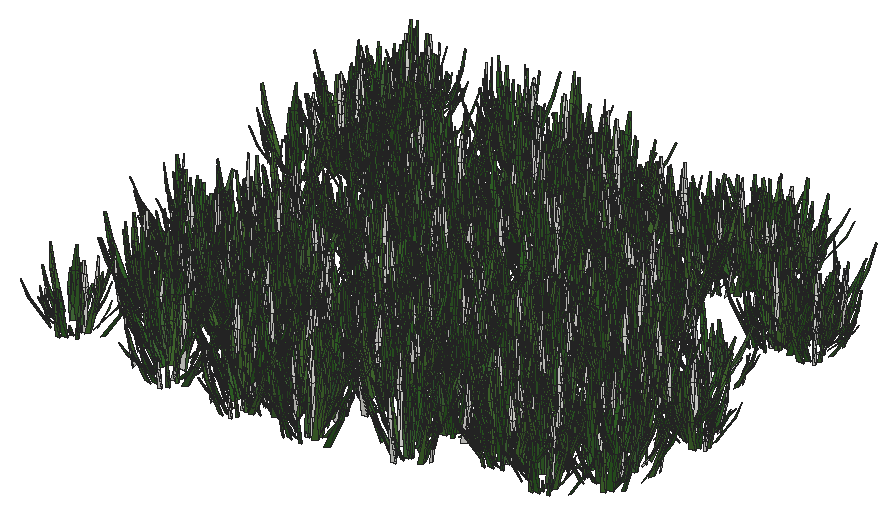
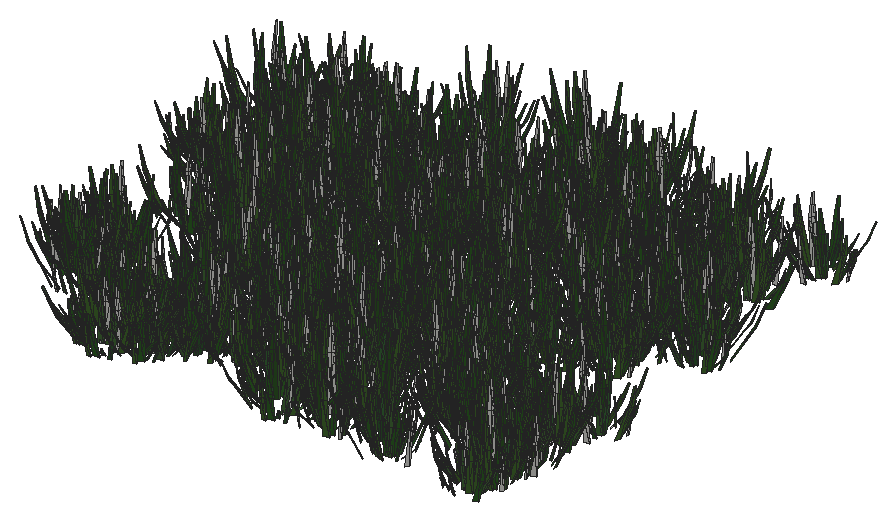
# SketchUp Ruby script. Lengths in inches.
U = 1.inch
M = Sketchup.active_model
def pt(a) = Geom::Point3d.new(a.map { |v| v * U })
def face(e, loops, mat)
  f = e.add_face(loops[0].map { |a| pt(a) })
  loops[1..].each { |l| e.add_face(l.map { |a| pt(a) }).erase! }
  f.material = f.back_material = mat if mat
  f
end
# faces: each face lists its corners as indices into pts; further lists are holes
def faces(e, pts, list, mat = nil) = list.each { |f| face(e, (f[0].is_a?(Array) ? f : [f]).map { |l| l.map { |i| pts[i] } }, mat) }
# xy, xz, yz: faces in a plane at the given z, y or x. An outline is a flat list of corners, or four numbers for a rectangle; further outlines are holes
def ring(l) = l.size == 4 ? [[l[0], l[1]], [l[2], l[1]], [l[2], l[3]], [l[0], l[3]]] : l.each_slice(2).to_a
def flat(e, list, mat, &to3) = list.each { |f| face(e, (f[0].is_a?(Array) ? f : [f]).map { |l| ring(l).map { |u, v| to3.(u, v) } }, mat) }
def xy(e, z, list, mat = nil) = flat(e, list, mat) { |x, y| [x, y, z] }
def xz(e, y, list, mat = nil) = flat(e, list, mat) { |x, z| [x, y, z] }
def yz(e, x, list, mat = nil) = flat(e, list, mat) { |y, z| [x, y, z] }
def lines(e, pts, list) = list.each { |a, b| e.add_line(pt(pts[a]), pt(pts[b])) }
# prism: a flat outline (further loops are holes) pulled along v
def prism(e, loops, v, mat = nil)
  f = face(e, loops, mat); d = Geom::Vector3d.new(v.map { |x| x * U })
  f.pushpull(f.normal.samedirection?(d) ? d.length : -d.length)
end
def box(e, o, s, mat = nil) = prism(e, [[o, [o[0] + s[0], o[1], o[2]], [o[0] + s[0], o[1] + s[1], o[2]], [o[0], o[1] + s[1], o[2]]]], [0, 0, s[2]], mat)
def at(x, y, z, deg = 0) = Geom::Transformation.translation(pt([x, y, z])) * Geom::Transformation.rotation(ORIGIN, Z_AXIS, deg.degrees)
def axes(o, x, y, z) = Geom::Transformation.new([*x, 0, *y, 0, *z, 0, *pt(o).to_a, 1])
def part(name) = M.definitions.add(name)
# library, detail: a bought-in or finely detailed component or shape, given as its bounding box
def library(name, o, s) = part(name).tap { |d| box(d.entities, o, s) }
def detail(e, o, s) = box(e.add_group.entities, o, s)
def put(e, d, t, mat = nil) = e.add_instance(d, t).tap { |i| i.material = mat if mat }
def group(e, t, mat = nil) = e.add_group.tap { |g| g.transformation = t; g.material = mat if mat }.entities
root = M.entities
M.materials.add("Material1").color = [58, 110, 58]
M.materials.add("Material10").color = [48, 100, 38]
M.materials.add("Material3").color = [68, 110, 58]
M.materials.add("Material4").color = [48, 90, 38]
M.materials.add("Material5").color = [68, 110, 48]
M.materials.add("Material6").color = [48, 90, 48]
M.materials.add("Material8").color = [58, 90, 38]
M.materials.add("Material9").color = [68, 100, 58]
c1 = part("grass00")
p = [[-0.6875,0.15,0],[-0.56,0.08,5.52],[-0.04,0.03,2.76],[0.48,-0.02,0],[0.35,-0.02,5.52],[-0.1,-0.14,5.52],
  [-0.12,0.65,8.37],[-0.42,0.65,8.37]]
faces(c1.entities,p,[[0,1,2,3],[3,2,4],[1,5,2],[5,4,2],[1,6,5],[4,5,6],[7,6,1]])
c2 = part("Group16\#1")
put(c2.entities,c1,axes([1.44,-0.61,-0.01],[0.05352,0.12609,0],[-0.10704,0.04543,0.07239],[0.06664,-0.02828,0.11628]),"Material6")
put(c2.entities,c1,axes([0.76,-0.15,-0.01],[0.04676,0.24062,0],[-0.23162,0.04501,0.06642],[0.0652,-0.01267,0.23595]),"Material3")
put(c2.entities,c1,axes([0.79,0.01,-0.01],[-0.00606,0.34651,0],[-0.34381,-0.00602,0.0432],[0.04319,0.00076,0.34386]))
put(c2.entities,c1,axes([1,0.23,-0.01],[-0.07192,0.31144,0],[-0.28722,-0.06632,0.1236],[0.12043,0.02781,0.29478]),"Material5")
put(c2.entities,c1,axes([1.66,0.77,-0.01],[-0.13828,0.29651,0],[-0.21551,-0.1005,0.22471],[0.20365,0.09498,0.23779]),"Material10")
put(c2.entities,c1,axes([0.6875,0.52,-0.01],[-0.18126,0.24051,0],[-0.22746,-0.17142,0.09788],[0.07817,0.05891,0.28481]),"Material5")
put(c2.entities,c1,axes([0.68,0.78,-0.01],[-0.215,0.18688,0],[-0.12385,-0.14248,0.21334],[0.13995,0.16101,0.18878]),"Material3")
put(c2.entities,c1,axes([0.56,1,-0.01],[-0.13756,0.07624,0],[-0.06159,-0.11112,0.0927],[0.04494,0.08108,0.12705]),"Material5")
put(c2.entities,c1,axes([0.2,0.64,-0.01],[-0.23729,0.07254,0],[-0.05711,-0.18681,0.153],[0.04473,0.14632,0.19535]),"Material10")
put(c2.entities,c1,axes([0.0625,0.72,-0.01],[-0.28874,0.02525,0],[-0.02179,-0.24916,0.14647],[0.01276,0.14591,0.25012]),"Material3")
put(c2.entities,c1,axes([-0.08,0.62,-0.01],[-0.34089,-0.04187,0],[0.03255,-0.26504,0.216],[-0.02633,0.21439,0.26703]),"Material10")
put(c2.entities,c1,axes([-0.34,0.98,-0.01],[-0.14314,-0.0493,0],[0.04397,-0.12769,0.06843],[-0.02228,0.0647,0.13505]),"Material10")
put(c2.entities,c1,axes([-0.87,1.45,-0.01],[-0.23488,-0.14114,0],[0.13761,-0.22901,0.06087],[-0.03135,0.05217,0.26717]))
put(c2.entities,c1,axes([-0.72,0.77,-0.01],[-0.14208,-0.13251,0],[0.07209,-0.0773,0.16301],[-0.11118,0.11922,0.1057]),"Material10")
put(c2.entities,c1,axes([-0.62,0.43,-0.01],[-0.14845,-0.21203,0],[0.18654,-0.13061,0.12304],[-0.10079,0.07057,0.22772]),"Material3")
put(c2.entities,c1,axes([-0.68,0.29,-0.01],[-0.13639,-0.32136,0],[0.31723,-0.13464,0.05579],[-0.05136,0.0218,0.34462]),"Material4")
put(c2.entities,c1,axes([-0.64,0.125,-0.01],[-0.0458,-0.23569,0],[0.22124,-0.043,0.08276],[-0.08124,0.01579,0.22538]),"Material1")
put(c2.entities,c1,axes([-1.6,-0.03,-0.01],[0.00576,-0.32897,0],[0.27526,0.00482,0.18018],[-0.18015,-0.00315,0.2753]),"Material5")
put(c2.entities,c1,axes([-1.36,-0.31,-0.01],[0.05718,-0.24765,0],[0.18172,0.04196,0.17267],[-0.16825,-0.03885,0.1865]),"Material10")
put(c2.entities,c1,axes([-1.54,-0.72,-0.01],[0.06537,-0.14017,0],[0.13555,0.06321,0.03939],[-0.0357,-0.01665,0.14956]))
put(c2.entities,c1,axes([-1.19,-0.9,-0.01],[0.09597,-0.12735,0],[0.11214,0.08451,0.07557],[-0.06035,-0.04548,0.14042]),"Material9")
put(c2.entities,c1,axes([-0.47,-0.54,-0.01],[0.11588,-0.10072,0],[0.0618,0.0711,0.12124],[-0.07953,-0.0915,0.0942]))
put(c2.entities,c1,axes([-0.47,-0.84,-0.01],[0.11927,-0.0661,0],[0.06603,0.11913,0.00646],[-0.00313,-0.00565,0.13621]),"Material5")
put(c2.entities,c1,axes([-0.38,-1.24,-0.01],[0.28037,-0.08571,0],[0.0618,0.20215,0.20315],[-0.05939,-0.19428,0.21139]),"Material9")
put(c2.entities,c1,axes([-0.06,-0.66,-0.01],[0.22719,-0.01987,0],[0.01247,0.14255,0.17758],[-0.01547,-0.17691,0.1431]),"Material8")
put(c2.entities,c1,axes([0.11,-0.89,-0.01],[0.14882,0.01828,0],[-0.01058,0.08611,0.12229],[0.01491,-0.12138,0.08676]),"Material6")
put(c2.entities,c1,axes([0.25,-0.72,-0.01],[0.20481,0.07053,0],[-0.06206,0.18022,0.10291],[0.03351,-0.0973,0.1906]),"Material6")
put(c2.entities,c1,axes([0.85,-1.42,-0.01],[0.16481,0.09904,0],[-0.09472,0.15762,0.05616],[0.02893,-0.04814,0.18389]),"Material5")
put(c2.entities,c1,axes([1.01,-1.09,-0.01],[0.21858,0.20385,0],[-0.17495,0.1876,0.15339],[0.10462,-0.11218,0.25652]),"Material10")
put(c2.entities,c1,axes([1.01,-0.71,-0.01],[0.08733,0.12473,0],[-0.06445,0.04512,0.13037],[0.1068,-0.07477,0.07867]),"Material6")
c3 = part("Group15\#1")
put(c3.entities,c2,at(0,0,0))
c4 = part("3darcstudiotree_grass00\#1")
put(c4.entities,c3,at(0,0,0))
put(root,c4,axes([316.35,97.13,0.25],[0.80132,-0.79526,0],[0.85381,0.59267,-0.02296],[0.02904,0.02016,1.8355]))
put(root,c4,axes([311.95,97.03,0.25],[0.12403,0.97719,0],[-0.92314,0.08072,-0.01763],[-0.03038,0.00266,1.60818]))
put(root,c4,axes([306.93,97.28,0.25],[0.20724,0.95588,0],[-1.27061,0.18977,-0.03105],[-0.03558,0.00531,1.50318]))
put(root,c4,axes([299.84,98.125,0.25],[0.90774,-0.36682,0],[0.49789,0.84879,-0.02466],[0.01422,0.02424,1.49812]))
put(root,c4,axes([313.64,97.92,0.25],[0.71273,0.60572,0],[-0.70706,0.57314,-0.01838],[-0.02206,0.01788,1.65818]))
put(root,c4,axes([321.96,98.48,0.25],[-0.85719,0.37482,0],[-0.44623,-0.70302,-0.01732],[-0.0161,-0.02536,1.90951]))
put(root,c4,axes([305.42,99.13,0.25],[1.00849,0.25736,0],[-0.35211,0.95054,-0.02064],[-0.00744,0.02009,1.46981]))
put(root,c4,axes([310.03,99.36,0.25],[0.41909,-0.86527,0],[1.14973,0.38363,-0.01772],[0.02372,0.00791,1.7874]))
put(root,c4,axes([315.09,99.53,0.25],[-0.98897,0.46793,0],[-0.61487,-0.89525,-0.01918],[-0.01379,-0.02007,1.80194]))
put(root,c4,axes([329.375,100.51,0.25],[1.05308,-0.43732,0],[0.41642,0.6908,-0.01525],[0.01172,0.01944,1.59832]))
put(root,c4,axes([326.36,101.1875,0.25],[0.78883,-0.48342,0],[0.67697,0.76099,-0.02283],[0.01727,0.01941,1.4512]))
put(root,c4,axes([303.67,101.62,0.25],[1.18479,-0.24576,0],[0.30744,1.02105,-0.03338],[0.00879,0.02919,1.37691]))
put(root,c4,axes([321.91,101.61,0.25],[-1.05079,-0.61219,0],[0.56436,-0.66733,-0.02484],[0.02413,-0.02854,1.66133]))
put(root,c4,axes([308.4375,101.85,0.25],[1.16137,-0.01703,0],[0.0221,1.03814,-0.02875],[0.00063,0.02974,1.55972]))
put(root,c4,axes([303.02,101.74,0.25],[-0.72355,-0.65418,0],[0.95278,-0.72597,-0.02326],[0.02414,-0.01839,1.82249]))
put(root,c4,axes([313.32,101.96,0.25],[0.32014,-0.85505,0],[1.06307,0.2742,-0.02169],[0.02869,0.0074,1.54236]))
put(root,c4,axes([325.75,102.07,0.25],[1.03078,-0.2005,0],[0.29521,1.04552,-0.02268],[0.00619,0.02191,1.5468]))
put(root,c4,axes([317.88,101.84,0.25],[-0.934,0.44634,0],[-0.64253,-0.92624,-0.0199],[-0.01289,-0.01859,1.67187]))
put(root,c4,axes([311.94,102.48,0.25],[-0.6646,-0.67167,0],[0.74435,-0.50738,-0.021],[0.02364,-0.01611,1.40308]))
put(root,c4,axes([301.47,102.32,0.25],[-0.81371,0.66575,0],[-0.86342,-0.727,-0.01243],[-0.01253,-0.01055,1.76595]))
put(root,c4,axes([331.54,102.84,0.25],[1.28074,0.0617,0],[-0.0694,0.99245,-0.0212],[-0.00202,0.02883,1.96575]))
put(root,c4,axes([324.94,103.13,0.25],[0.07007,-0.79845,0],[0.91239,0.05516,-0.00937],[0.0198,0.0012,1.93766]))
put(root,c4,axes([319.48,103.07,0.25],[-0.36362,-0.73138,0],[1.12762,-0.38622,-0.01762],[0.01979,-0.00678,1.48208]))
put(root,c4,axes([327.05,102.92,0.25],[-0.4787,0.65235,0],[-0.88098,-0.44536,-0.03041],[-0.03325,-0.01681,1.3205]))
put(root,c4,axes([308.77,103.05,0.25],[-1.08604,-0.15157,0],[0.17672,-0.87228,-0.0114],[0.0035,-0.01728,1.97478]))
put(root,c4,axes([328.02,103.05,0.25],[-0.16041,0.91007,0],[-0.94249,-0.11444,-0.02144],[-0.04347,-0.00528,1.9513]))
put(root,c4,axes([304.47,103.25,0.25],[-0.94592,0.10903,0],[-0.1657,-0.99036,-0.02154],[-0.00353,-0.02108,1.4342]))
put(root,c4,axes([313.27,103.47,0.25],[-0.88718,-0.16403,0],[0.21188,-0.78948,-0.02543],[0.00915,-0.03409,1.61262]))
put(root,c4,axes([317.96,104.16,0.25],[0.65668,-0.79697,0],[0.79285,0.45005,-0.02882],[0.03521,0.01999,1.42183]))
put(root,c4,axes([322.01,104.29,0.25],[1.1345,0.2801,0],[-0.33208,0.9266,-0.03162],[-0.0104,0.02903,1.3441]))
put(root,c4,axes([302.77,104.28,0.25],[0.93252,0.18888,0],[-0.22324,0.75929,-0.01459],[-0.00645,0.02194,1.75568]))
put(root,c4,axes([315.06,104.44,0.25],[1.27135,0.10554,0],[-0.11776,0.97731,-0.02551],[-0.00318,0.02637,1.48132]))
put(root,c4,axes([305.96,104.14,0.25],[-0.95929,-0.15943,0],[0.24233,-1.00448,-0.02406],[0.00588,-0.02436,1.53532]))
put(root,c4,axes([304.3,104.21,0.25],[0.36677,0.87584,0],[-0.8672,0.25018,-0.01128],[-0.02111,0.00609,1.81963]))
put(root,c4,axes([316.33,104.4,0.25],[0.63898,0.91689,0],[-1.0111,0.48542,-0.02506],[-0.03395,0.0163,1.82822]))
put(root,c4,axes([308.27,104.79,0.25],[-0.23441,-0.84252,0],[0.89566,-0.17167,-0.0292],[0.04766,-0.00914,1.53984]))
put(root,c4,axes([331.91,104.58,0.25],[-1.08025,0.12081,0],[-0.14812,-0.9124,-0.01091],[-0.00245,-0.01509,1.8656]))
put(root,c4,axes([311.97,104.98,0.25],[-1.17861,0.11572,0],[-0.13809,-0.96888,-0.02284],[-0.00331,-0.0232,1.44864]))
put(root,c4,axes([309.13,105.45,0.25],[-0.68321,-0.72872,0],[0.78352,-0.50606,-0.01663],[0.02499,-0.01614,1.89037]))
put(root,c4,axes([328.33,105.7,0.25],[0.40907,-0.67881,0],[0.97262,0.40378,-0.01805],[0.02352,0.00976,1.58457]))
put(root,c4,axes([303.86,105.63,0.25],[0.86846,0.22562,0],[-0.28927,0.76707,-0.01935],[-0.01148,0.03043,1.92273]))
put(root,c4,axes([322.75,105.79,0.25],[0.97724,-0.26245,0],[0.36108,0.9262,-0.01717],[0.0067,0.0172,1.48777]))
put(root,c4,axes([319.73,105.9,0.25],[0.96998,-0.05804,0],[0.06668,0.76779,-0.00836],[0.00128,0.01473,1.97523]))
put(root,c4,axes([316.75,105.83,0.25],[0.12117,0.83819,0],[-0.93224,0.09284,-0.01784],[-0.034,0.00339,1.80168]))
put(root,c4,axes([309.8125,105.86,0.25],[0.04694,1.0652,0],[-1.26088,0.03828,-0.0182],[-0.02086,0.00063,1.44668]))
put(root,c4,axes([326.38,106.08,0.25],[-0.28901,0.78465,0],[-1.0714,-0.27186,-0.0271],[-0.04002,-0.01015,1.72974]))
put(root,c4,axes([305.92,106.65,0.25],[0.07107,0.86763,0],[-1.08123,0.06101,-0.02807],[-0.03406,0.00192,1.3177]))
put(root,c4,axes([325.18,106.91,0.25],[-1.06982,0.08364,0],[-0.10313,-0.90868,-0.0202],[-0.00337,-0.02969,1.95637]))
put(root,c4,axes([317.59,107.38,0.25],[0.86287,-0.53565,0],[0.7402,0.82143,-0.02614],[0.01879,0.02086,1.48366]))
put(root,c4,axes([300.78,107.27,0.25],[1.16448,0.38507,0],[-0.42835,0.89237,-0.01606],[-0.00795,0.01656,1.54782]))
put(root,c4,axes([330.03,107.22,0.25],[0.60099,0.7227,0],[-0.87959,0.5039,-0.02215],[-0.0291,0.01667,1.70619]))
put(root,c4,axes([318.74,107.37,0.25],[-0.84677,-0.53059,0],[0.70417,-0.77417,-0.01411],[0.01233,-0.01356,1.69584]))
put(root,c4,axes([308.43,107.44,0.25],[-0.07251,0.86254,0],[-1.06517,-0.06169,-0.02357],[-0.034,-0.00197,1.54387]))
put(root,c4,axes([299.66,107.88,0.25],[0.62341,-0.65045,0],[0.81136,0.53571,-0.01848],[0.02058,0.01359,1.47553]))
put(root,c4,axes([320.87,108.25,0.25],[0.32381,0.70798,0],[-1.1928,0.37583,-0.02635],[-0.03281,0.01034,1.69955]))
put(root,c4,axes([316.57,108.31,0.25],[0.65479,0.79637,0],[-0.75973,0.43034,-0.01403],[-0.02494,0.01413,1.97952]))
put(root,c4,axes([313.28,108.45,0.25],[-0.31977,-0.73816,0],[0.97929,-0.29225,-0.0171],[0.02773,-0.00828,1.79343]))
put(root,c4,axes([312.07,108.25,0.25],[0.23878,1.03245,0],[-1.19555,0.19048,-0.02457],[-0.03165,0.00504,1.59681]))
put(root,c4,axes([303.11,108.54,0.25],[-0.25504,0.90723,0],[-0.99851,-0.19338,-0.02125],[-0.02713,-0.00525,1.34411]))
put(root,c4,axes([305.28,108.6,0.25],[-0.52673,0.64023,0],[-0.75004,-0.4251,-0.01899],[-0.03039,-0.01722,1.75992]))
put(root,c4,axes([323.56,109.13,0.25],[1.0339,-0.45076,0],[0.45476,0.71859,-0.02304],[0.01955,0.0309,1.78453]))
put(root,c4,axes([321.25,109.39,0.25],[0.04633,-0.80855,0],[0.9767,0.03855,-0.0123],[0.02217,0.00088,1.7643]))
put(root,c4,axes([317.79,109.36,0.25],[-0.28741,-0.72638,0],[0.96366,-0.26268,-0.02104],[0.0287,-0.00782,1.45661]))
put(root,c4,axes([332.67,109.11,0.25],[-0.50829,0.70684,0],[-0.88646,-0.43915,-0.0186],[-0.02272,-0.01125,1.46845]))
put(root,c4,axes([299.2,109.625,0.25],[-1.10338,-0.30687,0],[0.31079,-0.76983,-0.02118],[0.01148,-0.02843,1.66873]))
put(root,c4,axes([331.375,109.95,0.25],[-0.28588,-0.97039,0],[1.21013,-0.2456,-0.03172],[0.03382,-0.00686,1.36741]))
put(root,c4,axes([327.19,109.6875,0.25],[-0.19365,0.85401,0],[-1.21133,-0.18922,-0.01956],[-0.02828,-0.00442,1.8138]))
put(root,c4,axes([311.23,109.73,0.25],[-0.46557,0.88149,0],[-0.85697,-0.31181,-0.01229],[-0.02382,-0.00867,1.9803]))
put(root,c4,axes([316.24,110.5,0.25],[1.27169,-0.1612,0],[0.14546,0.79054,-0.02943],[0.00699,0.03801,1.51666]))
put(root,c4,axes([326.95,110.93,0.25],[-0.95819,-0.35748,0],[0.36939,-0.68208,-0.02079],[0.01525,-0.02816,1.61237]))
put(root,c4,axes([305.45,110.91,0.25],[-1.11893,-0.19294,0],[0.25521,-1.01964,-0.02537],[0.00751,-0.03001,1.82613]))
put(root,c4,axes([328.55,111.28,0.25],[0.57634,-0.70266,0],[0.90577,0.51181,-0.01892],[0.02488,0.01406,1.74337]))
put(root,c4,axes([323.92,111.11,0.25],[0.80339,0.50827,0],[-0.58384,0.63574,-0.01463],[-0.01601,0.01743,1.73802]))
put(root,c4,axes([317.8,110.97,0.25],[-1.24958,0.10274,0],[-0.09107,-0.76308,-0.0174],[-0.0032,-0.02684,1.72585]))
put(root,c4,axes([302.15,111.21,0.25],[-0.54044,-0.83323,0],[0.96155,-0.42964,-0.02018],[0.03177,-0.01419,1.95264]))
put(root,c4,axes([320.93,111.87,0.25],[0.88102,0.19888,0],[-0.2921,0.89141,-0.02379],[-0.00841,0.02566,1.49895]))
put(root,c4,axes([311.74,111.98,0.25],[0.91654,0.42489,0],[-0.49728,0.73898,-0.02091],[-0.01555,0.02311,1.55496]))
put(root,c4,axes([303.62,111.8125,0.25],[-0.78623,0.83967,0],[-0.77178,-0.49784,-0.03149],[-0.03404,-0.02196,1.33797]))
put(root,c4,axes([321.875,112.1,0.25],[0.58794,0.7169,0],[-0.77809,0.43961,-0.02533],[-0.03533,0.01996,1.58831]))
put(root,c4,axes([324.26,112.26,0.25],[0.92637,0.60353,0],[-0.62404,0.65986,-0.02005],[-0.0228,0.02411,1.86077]))
put(root,c4,axes([326.75,112.17,0.25],[-0.61592,0.73394,0],[-0.79423,-0.45916,-0.01437],[-0.02338,-0.01352,1.91898]))
put(root,c4,axes([312.96,112.51,0.25],[-0.69305,-0.66666,0],[0.88309,-0.63244,-0.03179],[0.0275,-0.01969,1.33245]))
put(root,c4,axes([302.39,112.93,0.25],[0.8253,-0.5081,0],[0.63121,0.70631,-0.02804],[0.02455,0.02747,1.55696]))
put(root,c4,axes([321.98,113.01,0.25],[0.58294,0.61529,0],[-0.97292,0.635,-0.01217],[-0.01408,0.00919,1.82194]))
put(root,c4,axes([319.36,113.43,0.25],[1.20286,-0.08126,0],[0.0966,0.98504,-0.02372],[0.0024,0.02445,1.48337]))
put(root,c4,axes([307.25,113.15,0.25],[-0.95152,-0.19631,0],[0.29747,-0.99332,-0.01735],[0.00577,-0.01928,1.70162]))
put(root,c4,axes([317.95,113.44,0.25],[1.03718,0.55321,0],[-0.70077,0.90509,-0.03131],[-0.01945,0.02512,1.48921]))
put(root,c4,axes([314.17,113.61,0.25],[-0.70254,0.68427,0],[-0.92407,-0.65358,-0.01912],[-0.01621,-0.01147,1.35238]))
put(root,c4,axes([312.12,113.72,0.25],[-0.97108,0.42527,0],[-0.49629,-0.7807,-0.01893],[-0.01139,-0.01792,1.37131]))
put(root,c4,axes([315.07,114.3125,0.25],[-0.10669,0.80768,0],[-1.01448,-0.09232,-0.02456],[-0.04084,-0.00372,1.70727]))
put(root,c4,axes([305.27,114.47,0.25],[-1.01459,-0.57502,0],[0.51409,-0.62489,-0.01838],[0.02057,-0.025,1.80866]))
put(root,c4,axes([329.32,114.73,0.25],[-1.14951,0.07107,0],[-0.07117,-0.79306,-0.0204],[-0.00216,-0.02409,1.3669]))
put(root,c4,axes([309.68,114.86,0.25],[-1.00145,-0.49535,0],[0.54618,-0.7607,-0.01663],[0.01553,-0.02163,1.94585]))
put(root,c4,axes([320.8,114.99,0.25],[-0.59135,0.86757,0],[-0.96172,-0.45159,-0.02589],[-0.02858,-0.01342,1.40149]))
put(root,c4,axes([324.91,115.6,0.25],[-0.35506,-0.69296,0],[1.04061,-0.36732,-0.01791],[0.02769,-0.00977,1.89984]))
put(root,c4,axes([310.39,115.61,0.25],[-1.10357,-0.1539,0],[0.16872,-0.83348,-0.01654],[0.00511,-0.02523,1.89711]))
put(root,c4,axes([306.85,115.91,0.25],[0.53466,0.61624,0],[-0.7851,0.46925,-0.02117],[-0.0301,0.01799,1.69559]))
put(root,c4,axes([316.21,117.12,0.25],[1.01453,-0.24669,0],[0.31532,0.89333,-0.01036],[0.00503,0.01424,1.93559]))
put(root,c4,axes([308.36,116.89,0.25],[0.55253,0.95891,0],[-0.94558,0.37535,-0.02212],[-0.03718,0.01476,1.95299]))
put(root,c4,axes([312.83,117.13,0.25],[-0.83676,-0.36548,0],[0.46586,-0.73476,-0.01604],[0.0142,-0.0224,1.9024]))
put(root,c4,axes([322.05,117.04,0.25],[-0.41283,0.85285,0],[-1.03697,-0.3458,-0.02547],[-0.02931,-0.00978,1.38631]))
put(root,c4,axes([323.68,117.32,0.25],[-0.75666,-0.75068,0],[0.85742,-0.59539,-0.01878],[0.02166,-0.01504,1.68146]))
put(root,c4,axes([323.67,117.93,0.25],[-1.1416,0.45714,0],[-0.45611,-0.78467,-0.02532],[-0.01721,-0.02961,1.64221]))
put(root,c4,axes([311.72,118.4,0.25],[1.15172,0.48664,0],[-0.57188,0.9324,-0.01612],[-0.0094,0.01532,1.61949]))
put(root,c4,axes([298.58,118.59,0.25],[1.04476,-0.17024,0],[0.22274,0.94168,-0.02697],[0.00719,0.03039,1.59996]))
put(root,c4,axes([305.64,118.59,0.25],[1.14989,-0.07767,0],[0.09108,0.92892,-0.01977],[0.00228,0.02329,1.59866]))
put(root,c4,axes([315.29,118.28,0.25],[-1.09908,0.39917,0],[-0.45844,-0.86957,-0.02625],[-0.01345,-0.02552,1.46233]))
put(root,c4,axes([313.1,119.18,0.25],[0.11479,-0.84282,0],[1.27851,0.11996,-0.01256],[0.01851,0.00174,1.90836]))
put(root,c4,axes([329.55,119.66,0.25],[0.60422,-0.56041,0],[0.75524,0.56096,-0.01984],[0.02658,0.01974,1.82222]))
put(root,c4,axes([308.93,119.32,0.25],[-0.58539,0.70478,0],[-0.86705,-0.49612,-0.02321],[-0.03085,-0.01765,1.70026]))
put(root,c4,axes([302.13,119.61,0.25],[-0.65603,-0.5606,0],[0.71497,-0.57639,-0.02073],[0.02312,-0.01864,1.5494]))
put(root,c4,axes([318.17,119.78,0.25],[0.93409,0.02419,0],[-0.03025,0.8046,-0.01718],[-0.00104,0.02764,1.88076]))
put(root,c4,axes([320.52,119.48,0.25],[-0.84085,0.70874,0],[-0.79442,-0.64929,-0.02428],[-0.02062,-0.01685,1.32917]))
put(root,c4,axes([319.37,119.6875,0.25],[-1.23523,-0.20438,0],[0.23939,-0.99669,-0.01918],[0.00583,-0.02427,1.90358]))
put(root,c4,axes([306.81,119.81,0.25],[-0.97997,0.02414,0],[-0.0316,-0.88394,-0.02538],[-0.00123,-0.03444,1.74242]))
put(root,c4,axes([314.81,119.92,0.25],[-0.98547,0.08818,0],[-0.114,-0.87772,-0.01956],[-0.00389,-0.02997,1.97453]))
put(root,c4,axes([315.88,120.65,0.25],[-0.74381,-0.67773,0],[0.74414,-0.56262,-0.02128],[0.03052,-0.02307,1.95268]))
put(root,c4,axes([331.53,120.43,0.25],[-0.33686,0.97485,0],[-1.05069,-0.25012,-0.02925],[-0.035,-0.00833,1.36051]))
put(root,c4,axes([299.59,120.53,0.25],[-0.38322,0.78723,0],[-0.97311,-0.32634,-0.02451],[-0.03595,-0.01205,1.66036]))
put(root,c4,axes([311.58,121.01,0.25],[1.04545,-0.31007,0],[0.38584,0.89621,-0.0155],[0.00909,0.02111,1.9985]))
put(root,c4,axes([305.78,120.57,0.25],[-1.03866,0.55303,0],[-0.58818,-0.76101,-0.01729],[-0.01396,-0.01807,1.62898]))
put(root,c4,axes([329.9,120.87,0.25],[-0.56024,-0.60752,0],[0.84978,-0.53985,-0.02737],[0.02644,-0.0168,1.30175]))
put(root,c4,axes([322.81,121.34,0.25],[-0.20461,-1.01308,0],[1.09619,-0.15252,-0.02808],[0.04178,-0.00581,1.67665]))
put(root,c4,axes([317.2,121.7,0.25],[-0.39916,-0.82921,0],[0.85209,-0.28257,-0.01431],[0.02515,-0.00834,1.73701]))
put(root,c4,axes([331.16,121.75,0.25],[0.56786,0.62975,0],[-0.85948,0.53391,-0.0157],[-0.01883,0.0117,1.60759]))
put(root,c4,axes([299.71,122.23,0.25],[0.96163,0.13462,0],[-0.17847,0.87825,-0.03005],[-0.00719,0.03537,1.54341]))
put(root,c4,axes([305.75,122.15,0.25],[0.64763,0.68012,0],[-0.83997,0.55101,-0.02315],[-0.02789,0.0183,1.64391]))
put(root,c4,axes([329.375,123.1,0.25],[-0.80096,-0.8493,0],[0.99431,-0.64599,-0.01534],[0.01647,-0.0107,1.72134]))
put(root,c4,axes([304,123.26,0.25],[-0.765,-0.40628,0],[0.48643,-0.63097,-0.02395],[0.01995,-0.02588,1.39534]))
put(root,c4,axes([323.95,123.3,0.25],[0.60457,0.83299,0],[-1.11328,0.55663,-0.01693],[-0.01785,0.00893,1.59984]))
put(root,c4,axes([299.37,123.84,0.25],[1.11523,0.33303,0],[-0.32321,0.74562,-0.01256],[-0.00811,0.01871,1.82155]))
put(root,c4,axes([320.97,123.63,0.25],[-1.04008,0.60418,0],[-0.584,-0.69257,-0.01309],[-0.01384,-0.01641,1.87779]))
put(root,c4,axes([310.74,124.36,0.25],[1.05892,0.30103,0],[-0.31137,0.75455,-0.02009],[-0.01183,0.02866,1.7458]))
put(root,c4,axes([301.47,124.4375,0.25],[1.10584,-0.01819,0],[0.01997,0.83675,-0.01855],[0.00071,0.02956,1.93628]))
put(root,c4,axes([313.46,124.1875,0.25],[-0.35579,0.71591,0],[-0.99425,-0.3404,-0.01866],[-0.02496,-0.00855,1.55626]))
put(root,c4,axes([317.9375,124.21,0.25],[-0.26469,0.96066,0],[-1.07431,-0.20391,-0.0233],[-0.03262,-0.00619,1.58282]))
put(root,c4,axes([311.8125,124.46,0.25],[-0.77916,-0.56674,0],[0.62456,-0.59153,-0.01406],[0.01734,-0.01643,1.77353]))
put(root,c4,axes([323.98,124.81,0.25],[0.1732,-1.02001,0],[1.12224,0.13128,-0.02402],[0.03864,0.00452,1.84088]))
put(root,c4,axes([299.6,124.8125,0.25],[0.68497,-0.50206,0],[0.63773,0.59939,-0.01409],[0.01592,0.01496,1.64399]))
put(root,c4,axes([314.68,124.65,0.25],[-0.32676,0.95361,0],[-0.99184,-0.23413,-0.01558],[-0.02763,-0.00652,1.90128]))
put(root,c4,axes([324.88,125.12,0.25],[0.85231,-0.62721,0],[0.75745,0.70908,-0.03392],[0.02612,0.02445,1.32537]))
put(root,c4,axes([320.56,124.89,0.25],[-1.03128,-0.47774,0],[0.62196,-0.92493,-0.0179],[0.01113,-0.01655,1.62858]))
put(root,c4,axes([308.2,125.47,0.25],[-0.07037,0.86768,0],[-1.21376,-0.06781,-0.01753],[-0.02701,-0.00151,1.87889]))
put(root,c4,axes([299.57,126.26,0.25],[0.46964,-0.66633,0],[0.84807,0.41178,-0.02347],[0.0398,0.01933,1.9305]))
put(root,c4,axes([321.86,126.09,0.25],[-0.73814,-0.67676,0],[0.90122,-0.67715,-0.01753],[0.01583,-0.01189,1.48083]))
put(root,c4,axes([310,126.8125,0.25],[0.57659,-0.88321,0],[0.9737,0.43791,-0.00988],[0.01481,0.00666,1.88737]))
put(root,c4,axes([322.63,126.91,0.25],[-1.02748,0.04697,0],[-0.06451,-0.97215,-0.02509],[-0.00158,-0.02386,1.34616]))
put(root,c4,axes([305.72,127.21,0.25],[0.74006,0.53571,0],[-0.84796,0.80699,-0.01764],[-0.01569,0.01494,1.74631]))
put(root,c4,axes([325.04,127.17,0.25],[-0.68552,0.53333,0],[-0.82392,-0.72956,-0.02311],[-0.0182,-0.01611,1.38694]))
put(root,c4,axes([313.18,127.25,0.25],[-1.19758,0.40343,0],[-0.4274,-0.87403,-0.01879],[-0.00914,-0.01869,1.46955]))
put(root,c4,axes([300.02,127.44,0.25],[-0.41539,0.86117,0],[-0.90402,-0.3004,-0.01826],[-0.02563,-0.00852,1.47196]))
put(root,c4,axes([324.33,127.61,0.25],[-1.08048,0.47938,0],[-0.57091,-0.88647,-0.02635],[-0.01425,-0.02213,1.3895]))
